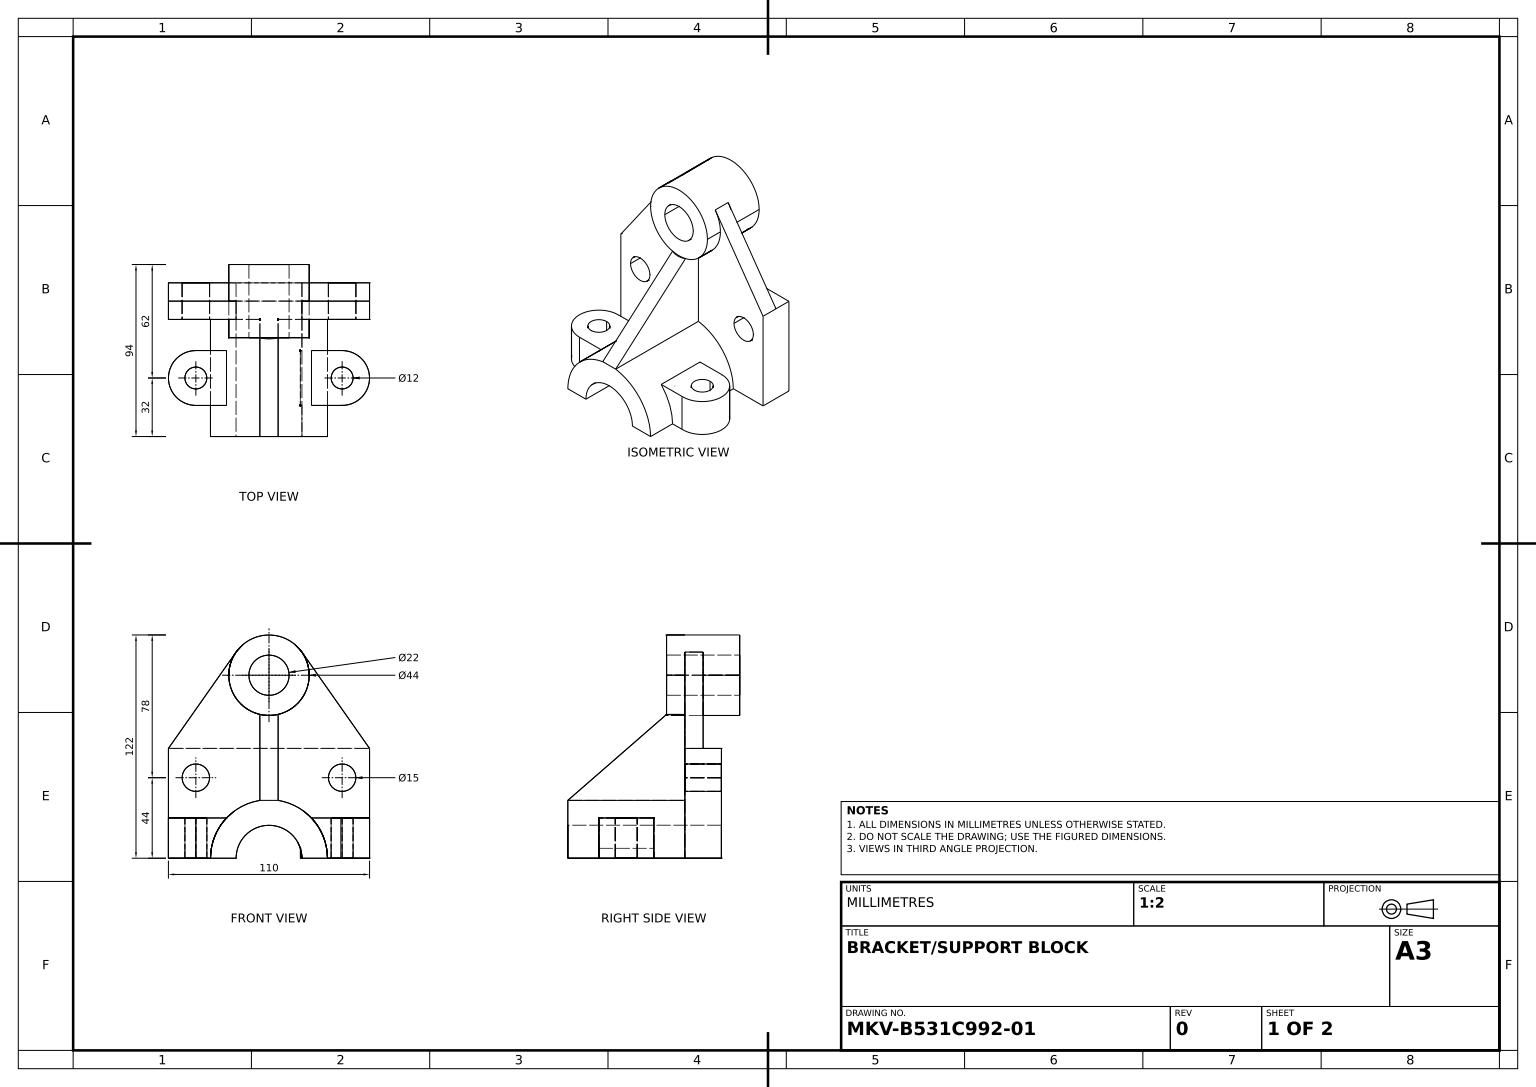
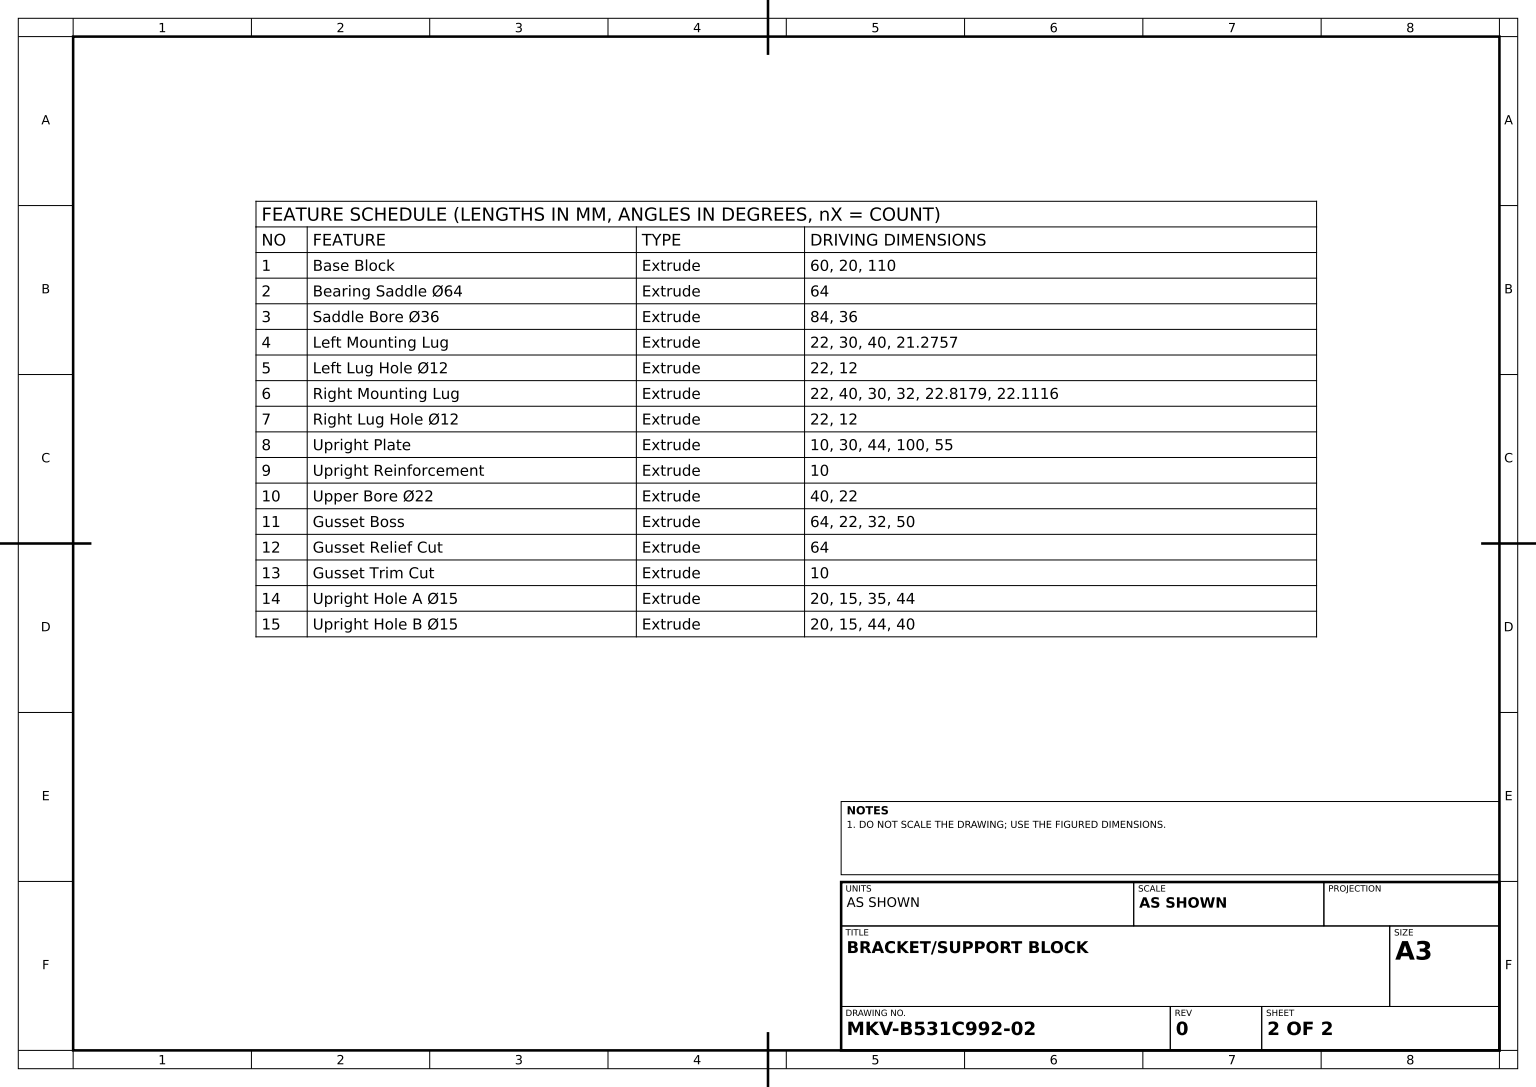
ISO-10303-21;
HEADER;
FILE_DESCRIPTION((''),'2;1');
FILE_NAME('','',(''),(''),'','','');
FILE_SCHEMA(('AUTOMOTIVE_DESIGN'));
ENDSEC;
DATA;
#1=APPLICATION_CONTEXT('');
#2=PRODUCT_CONTEXT('',#1,'mechanical');
#3=PRODUCT('','','',(#2));
#4=PRODUCT_DEFINITION_FORMATION('','',#3);
#5=PRODUCT_DEFINITION_CONTEXT('',#1,'design');
#6=PRODUCT_DEFINITION('','',#4,#5);
#7=PRODUCT_DEFINITION_SHAPE('','',#6);
#8=(LENGTH_UNIT()NAMED_UNIT(*)SI_UNIT(.MILLI.,.METRE.));
#9=(NAMED_UNIT(*)PLANE_ANGLE_UNIT()SI_UNIT($,.RADIAN.));
#10=(NAMED_UNIT(*)SI_UNIT($,.STERADIAN.)SOLID_ANGLE_UNIT());
#11=UNCERTAINTY_MEASURE_WITH_UNIT(LENGTH_MEASURE(1.E-05),#8,'distance_accuracy_value','');
#12=(GEOMETRIC_REPRESENTATION_CONTEXT(3)GLOBAL_UNCERTAINTY_ASSIGNED_CONTEXT((#11))GLOBAL_UNIT_ASSIGNED_CONTEXT((#8,#9,#10))REPRESENTATION_CONTEXT('',''));
#13=CARTESIAN_POINT('',(17.182133,5.364167,17.));
#14=VERTEX_POINT('',#13);
#15=CARTESIAN_POINT('',(17.182133,0.,17.));
#16=VERTEX_POINT('',#15);
#17=CARTESIAN_POINT('',(17.182133,22.,17.));
#18=DIRECTION('',(0.,-1.,0.));
#19=VECTOR('',#18,1000.);
#20=LINE('',#17,#19);
#21=EDGE_CURVE('',#14,#16,#20,.T.);
#22=ORIENTED_EDGE('',*,*,#21,.F.);
#23=CARTESIAN_POINT('',(18.,0.,17.));
#24=VERTEX_POINT('',#23);
#25=CARTESIAN_POINT('',(0.,0.,17.));
#26=DIRECTION('',(0.,0.,-1.));
#27=DIRECTION('',(1.,0.,0.));
#28=AXIS2_PLACEMENT_3D('',#25,#26,#27);
#29=CIRCLE('',#28,18.);
#30=EDGE_CURVE('',#14,#24,#29,.T.);
#31=ORIENTED_EDGE('',*,*,#30,.T.);
#32=CARTESIAN_POINT('',(40.,0.,17.));
#33=DIRECTION('',(-1.,0.,0.));
#34=VECTOR('',#33,1000.);
#35=LINE('',#32,#34);
#36=EDGE_CURVE('',#24,#16,#35,.T.);
#37=ORIENTED_EDGE('',*,*,#36,.T.);
#38=EDGE_LOOP('',(#22,#31,#37));
#39=FACE_OUTER_BOUND('',#38,.T.);
#40=CARTESIAN_POINT('',(40.,22.,17.));
#41=DIRECTION('',(0.,0.,1.));
#42=AXIS2_PLACEMENT_3D('',#40,#41,#27);
#43=PLANE('',#42);
#44=ADVANCED_FACE('',(#39),#43,.F.);
#45=CARTESIAN_POINT('',(-32.,0.,64.));
#46=VERTEX_POINT('',#45);
#47=CARTESIAN_POINT('',(-32.,0.,47.));
#48=VERTEX_POINT('',#47);
#49=VECTOR('',#26,1000.);
#50=LINE('',#45,#49);
#51=EDGE_CURVE('',#46,#48,#50,.T.);
#52=ORIENTED_EDGE('',*,*,#51,.T.);
#53=CARTESIAN_POINT('',(-40.,0.,47.));
#54=VERTEX_POINT('',#53);
#55=CARTESIAN_POINT('',(-18.724275,0.,47.));
#56=VECTOR('',#27,1000.);
#57=LINE('',#55,#56);
#58=EDGE_CURVE('',#54,#48,#57,.T.);
#59=ORIENTED_EDGE('',*,*,#58,.F.);
#60=CARTESIAN_POINT('',(-40.,0.,17.));
#61=VERTEX_POINT('',#60);
#62=CARTESIAN_POINT('',(-40.,0.,32.));
#63=DIRECTION('',(0.,1.,0.));
#64=AXIS2_PLACEMENT_3D('',#62,#63,#41);
#65=CIRCLE('',#64,15.);
#66=EDGE_CURVE('',#61,#54,#65,.T.);
#67=ORIENTED_EDGE('',*,*,#66,.F.);
#68=CARTESIAN_POINT('',(-32.,0.,17.));
#69=VERTEX_POINT('',#68);
#70=LINE('',#60,#34);
#71=EDGE_CURVE('',#69,#61,#70,.T.);
#72=ORIENTED_EDGE('',*,*,#71,.F.);
#73=CARTESIAN_POINT('',(-32.,0.,0.));
#74=VERTEX_POINT('',#73);
#75=EDGE_CURVE('',#69,#74,#50,.T.);
#76=ORIENTED_EDGE('',*,*,#75,.T.);
#77=CARTESIAN_POINT('',(-55.,0.,0.));
#78=VERTEX_POINT('',#77);
#79=CARTESIAN_POINT('',(55.,0.,0.));
#80=LINE('',#79,#56);
#81=EDGE_CURVE('',#78,#74,#80,.T.);
#82=ORIENTED_EDGE('',*,*,#81,.F.);
#83=CARTESIAN_POINT('',(-55.,0.,-20.));
#84=VERTEX_POINT('',#83);
#85=VECTOR('',#41,1000.);
#86=LINE('',#77,#85);
#87=EDGE_CURVE('',#84,#78,#86,.T.);
#88=ORIENTED_EDGE('',*,*,#87,.F.);
#89=CARTESIAN_POINT('',(-18.,0.,-20.));
#90=VERTEX_POINT('',#89);
#91=LINE('',#83,#34);
#92=EDGE_CURVE('',#90,#84,#91,.T.);
#93=ORIENTED_EDGE('',*,*,#92,.F.);
#94=CARTESIAN_POINT('',(-18.,0.,64.));
#95=VERTEX_POINT('',#94);
#96=LINE('',#89,#85);
#97=EDGE_CURVE('',#90,#95,#96,.T.);
#98=ORIENTED_EDGE('',*,*,#97,.T.);
#99=LINE('',#45,#56);
#100=EDGE_CURVE('',#46,#95,#99,.T.);
#101=ORIENTED_EDGE('',*,*,#100,.F.);
#102=EDGE_LOOP('',(#52,#59,#67,#72,#76,#82,#88,#93,#98,#101));
#103=FACE_OUTER_BOUND('',#102,.T.);
#104=CARTESIAN_POINT('',(-40.,0.,26.));
#105=VERTEX_POINT('',#104);
#106=CARTESIAN_POINT('',(-40.,0.,38.));
#107=VERTEX_POINT('',#106);
#108=CIRCLE('',#64,6.);
#109=EDGE_CURVE('',#105,#107,#108,.T.);
#110=ORIENTED_EDGE('',*,*,#109,.T.);
#111=EDGE_CURVE('',#107,#105,#108,.T.);
#112=ORIENTED_EDGE('',*,*,#111,.T.);
#113=EDGE_LOOP('',(#110,#112));
#114=FACE_BOUND('',#113,.T.);
#115=CARTESIAN_POINT('',(0.,0.,0.));
#116=AXIS2_PLACEMENT_3D('',#115,#18,#26);
#117=PLANE('',#116);
#118=ADVANCED_FACE('',(#103,#114),#117,.T.);
#119=CARTESIAN_POINT('',(11.,100.,-30.));
#120=VERTEX_POINT('',#119);
#121=CARTESIAN_POINT('',(-11.,100.,-30.));
#122=VERTEX_POINT('',#121);
#123=CARTESIAN_POINT('',(0.,100.,-30.));
#124=AXIS2_PLACEMENT_3D('',#123,#41,#27);
#125=CIRCLE('',#124,11.);
#126=EDGE_CURVE('',#120,#122,#125,.T.);
#127=ORIENTED_EDGE('',*,*,#126,.F.);
#128=CARTESIAN_POINT('',(11.,100.,10.));
#129=VERTEX_POINT('',#128);
#130=LINE('',#119,#85);
#131=EDGE_CURVE('',#120,#129,#130,.T.);
#132=ORIENTED_EDGE('',*,*,#131,.T.);
#133=CARTESIAN_POINT('',(-11.,100.,10.));
#134=VERTEX_POINT('',#133);
#135=CARTESIAN_POINT('',(0.,100.,10.));
#136=AXIS2_PLACEMENT_3D('',#135,#41,#27);
#137=CIRCLE('',#136,11.);
#138=EDGE_CURVE('',#129,#134,#137,.T.);
#139=ORIENTED_EDGE('',*,*,#138,.T.);
#140=LINE('',#121,#85);
#141=EDGE_CURVE('',#122,#134,#140,.T.);
#142=ORIENTED_EDGE('',*,*,#141,.F.);
#143=EDGE_LOOP('',(#127,#132,#139,#142));
#144=FACE_OUTER_BOUND('',#143,.T.);
#145=CYLINDRICAL_SURFACE('',#124,11.);
#146=ADVANCED_FACE('',(#144),#145,.F.);
#147=CARTESIAN_POINT('',(17.182133,5.364167,47.));
#148=VERTEX_POINT('',#147);
#149=CARTESIAN_POINT('',(17.182133,0.,47.));
#150=VERTEX_POINT('',#149);
#151=CARTESIAN_POINT('',(17.182133,22.,47.));
#152=LINE('',#151,#19);
#153=EDGE_CURVE('',#148,#150,#152,.T.);
#154=ORIENTED_EDGE('',*,*,#153,.T.);
#155=CARTESIAN_POINT('',(18.,0.,46.999385));
#156=VERTEX_POINT('',#155);
#157=DIRECTION('',(0.999999717,0.,-0.000752449));
#158=VECTOR('',#157,1000.);
#159=LINE('',#149,#158);
#160=EDGE_CURVE('',#150,#156,#159,.T.);
#161=ORIENTED_EDGE('',*,*,#160,.T.);
#162=CARTESIAN_POINT('',(18.,1.822601,46.999385));
#163=CARTESIAN_POINT('',(17.725286,3.62438,46.999591));
#164=(BOUNDED_CURVE()B_SPLINE_CURVE(3,(#155,#162,#163,#147),.UNSPECIFIED.,.F.,.T.)B_SPLINE_CURVE_WITH_KNOTS((4,4),(3.141592654,3.444199156),.UNSPECIFIED.)CURVE()GEOMETRIC_REPRESENTATION_ITEM()RATIONAL_B_SPLINE_CURVE((1.,0.992383655,0.992383655,1.))REPRESENTATION_ITEM(''));
#165=EDGE_CURVE('',#156,#148,#164,.T.);
#166=ORIENTED_EDGE('',*,*,#165,.T.);
#167=EDGE_LOOP('',(#154,#161,#166));
#168=FACE_OUTER_BOUND('',#167,.T.);
#169=DIRECTION('',(-0.000752449,0.,-0.999999717));
#170=DIRECTION('',(-0.999999717,0.,0.000752449));
#171=AXIS2_PLACEMENT_3D('',#151,#169,#170);
#172=PLANE('',#171);
#173=ADVANCED_FACE('',(#168),#172,.F.);
#174=CARTESIAN_POINT('',(-40.,22.,47.));
#175=VERTEX_POINT('',#174);
#176=CARTESIAN_POINT('',(-23.2379,22.,47.));
#177=VERTEX_POINT('',#176);
#178=CARTESIAN_POINT('',(-18.724275,22.,47.));
#179=LINE('',#178,#56);
#180=EDGE_CURVE('',#175,#177,#179,.T.);
#181=ORIENTED_EDGE('',*,*,#180,.T.);
#182=CARTESIAN_POINT('',(-23.2379,22.,17.));
#183=VERTEX_POINT('',#182);
#184=CARTESIAN_POINT('',(-23.2379,22.,64.));
#185=LINE('',#184,#85);
#186=EDGE_CURVE('',#183,#177,#185,.T.);
#187=ORIENTED_EDGE('',*,*,#186,.F.);
#188=CARTESIAN_POINT('',(-40.,22.,17.));
#189=VERTEX_POINT('',#188);
#190=LINE('',#188,#34);
#191=EDGE_CURVE('',#183,#189,#190,.T.);
#192=ORIENTED_EDGE('',*,*,#191,.T.);
#193=CARTESIAN_POINT('',(-40.,22.,32.));
#194=AXIS2_PLACEMENT_3D('',#193,#63,#41);
#195=CIRCLE('',#194,15.);
#196=EDGE_CURVE('',#189,#175,#195,.T.);
#197=ORIENTED_EDGE('',*,*,#196,.T.);
#198=EDGE_LOOP('',(#181,#187,#192,#197));
#199=FACE_OUTER_BOUND('',#198,.T.);
#200=CARTESIAN_POINT('',(-40.,22.,26.));
#201=VERTEX_POINT('',#200);
#202=CARTESIAN_POINT('',(-40.,22.,38.));
#203=VERTEX_POINT('',#202);
#204=CIRCLE('',#194,6.);
#205=EDGE_CURVE('',#201,#203,#204,.T.);
#206=ORIENTED_EDGE('',*,*,#205,.F.);
#207=EDGE_CURVE('',#203,#201,#204,.T.);
#208=ORIENTED_EDGE('',*,*,#207,.F.);
#209=EDGE_LOOP('',(#206,#208));
#210=FACE_BOUND('',#209,.T.);
#211=PLANE('',#194);
#212=ADVANCED_FACE('',(#199,#210),#211,.T.);
#213=CARTESIAN_POINT('',(5.,78.575715,10.));
#214=VERTEX_POINT('',#213);
#215=CARTESIAN_POINT('',(22.,100.,10.));
#216=VERTEX_POINT('',#215);
#217=CIRCLE('',#136,22.);
#218=EDGE_CURVE('',#214,#216,#217,.T.);
#219=ORIENTED_EDGE('',*,*,#218,.T.);
#220=CARTESIAN_POINT('',(-22.,100.,10.));
#221=VERTEX_POINT('',#220);
#222=EDGE_CURVE('',#216,#221,#217,.T.);
#223=ORIENTED_EDGE('',*,*,#222,.T.);
#224=CARTESIAN_POINT('',(-5.,78.575715,10.));
#225=VERTEX_POINT('',#224);
#226=EDGE_CURVE('',#221,#225,#217,.T.);
#227=ORIENTED_EDGE('',*,*,#226,.T.);
#228=EDGE_CURVE('',#225,#214,#217,.T.);
#229=ORIENTED_EDGE('',*,*,#228,.T.);
#230=EDGE_LOOP('',(#219,#223,#227,#229));
#231=FACE_OUTER_BOUND('',#230,.T.);
#232=ORIENTED_EDGE('',*,*,#138,.F.);
#233=EDGE_CURVE('',#134,#129,#137,.T.);
#234=ORIENTED_EDGE('',*,*,#233,.F.);
#235=EDGE_LOOP('',(#232,#234));
#236=FACE_BOUND('',#235,.T.);
#237=PLANE('',#136);
#238=ADVANCED_FACE('',(#231,#236),#237,.T.);
#239=CARTESIAN_POINT('',(-55.,60.,-20.));
#240=VERTEX_POINT('',#239);
#241=LINE('',#239,#19);
#242=EDGE_CURVE('',#240,#84,#241,.T.);
#243=ORIENTED_EDGE('',*,*,#242,.F.);
#244=CARTESIAN_POINT('',(55.,60.,-20.));
#245=VERTEX_POINT('',#244);
#246=LINE('',#239,#34);
#247=EDGE_CURVE('',#245,#240,#246,.T.);
#248=ORIENTED_EDGE('',*,*,#247,.F.);
#249=CARTESIAN_POINT('',(55.,0.,-20.));
#250=VERTEX_POINT('',#249);
#251=LINE('',#244,#19);
#252=EDGE_CURVE('',#245,#250,#251,.T.);
#253=ORIENTED_EDGE('',*,*,#252,.T.);
#254=CARTESIAN_POINT('',(18.,0.,-20.));
#255=VERTEX_POINT('',#254);
#256=EDGE_CURVE('',#250,#255,#91,.T.);
#257=ORIENTED_EDGE('',*,*,#256,.T.);
#258=CARTESIAN_POINT('',(0.,0.,-20.));
#259=AXIS2_PLACEMENT_3D('',#258,#41,#27);
#260=CIRCLE('',#259,18.);
#261=EDGE_CURVE('',#255,#90,#260,.T.);
#262=ORIENTED_EDGE('',*,*,#261,.T.);
#263=ORIENTED_EDGE('',*,*,#92,.T.);
#264=EDGE_LOOP('',(#243,#248,#253,#257,#262,#263));
#265=FACE_OUTER_BOUND('',#264,.T.);
#266=CARTESIAN_POINT('',(-47.5,44.,-20.));
#267=VERTEX_POINT('',#266);
#268=CARTESIAN_POINT('',(-32.5,44.,-20.));
#269=VERTEX_POINT('',#268);
#270=CARTESIAN_POINT('',(-40.,44.,-20.));
#271=AXIS2_PLACEMENT_3D('',#270,#41,#27);
#272=CIRCLE('',#271,7.5);
#273=EDGE_CURVE('',#267,#269,#272,.T.);
#274=ORIENTED_EDGE('',*,*,#273,.T.);
#275=EDGE_CURVE('',#269,#267,#272,.T.);
#276=ORIENTED_EDGE('',*,*,#275,.T.);
#277=EDGE_LOOP('',(#274,#276));
#278=FACE_BOUND('',#277,.T.);
#279=CARTESIAN_POINT('',(47.5,44.,-20.));
#280=VERTEX_POINT('',#279);
#281=CARTESIAN_POINT('',(32.5,44.,-20.));
#282=VERTEX_POINT('',#281);
#283=CARTESIAN_POINT('',(40.,44.,-20.));
#284=AXIS2_PLACEMENT_3D('',#283,#41,#27);
#285=CIRCLE('',#284,7.5);
#286=EDGE_CURVE('',#280,#282,#285,.T.);
#287=ORIENTED_EDGE('',*,*,#286,.T.);
#288=EDGE_CURVE('',#282,#280,#285,.T.);
#289=ORIENTED_EDGE('',*,*,#288,.T.);
#290=EDGE_LOOP('',(#287,#289));
#291=FACE_BOUND('',#290,.T.);
#292=AXIS2_PLACEMENT_3D('',#239,#41,#27);
#293=PLANE('',#292);
#294=ADVANCED_FACE('',(#265,#278,#291),#293,.F.);
#295=ORIENTED_EDGE('',*,*,#131,.F.);
#296=EDGE_CURVE('',#122,#120,#125,.T.);
#297=ORIENTED_EDGE('',*,*,#296,.F.);
#298=ORIENTED_EDGE('',*,*,#141,.T.);
#299=ORIENTED_EDGE('',*,*,#233,.T.);
#300=EDGE_LOOP('',(#295,#297,#298,#299));
#301=FACE_OUTER_BOUND('',#300,.T.);
#302=ADVANCED_FACE('',(#301),#145,.F.);
#303=CARTESIAN_POINT('',(-5.,31.606961,64.));
#304=VERTEX_POINT('',#303);
#305=CARTESIAN_POINT('',(-5.,51.83632,40.742296));
#306=DIRECTION('',(0.,0.65627603,-0.754520889));
#307=VECTOR('',#306,1000.);
#308=LINE('',#305,#307);
#309=EDGE_CURVE('',#304,#225,#308,.T.);
#310=ORIENTED_EDGE('',*,*,#309,.F.);
#311=CARTESIAN_POINT('',(5.,31.606961,64.));
#312=VERTEX_POINT('',#311);
#313=CARTESIAN_POINT('',(-64.,31.606961,64.));
#314=LINE('',#313,#56);
#315=EDGE_CURVE('',#304,#312,#314,.T.);
#316=ORIENTED_EDGE('',*,*,#315,.T.);
#317=CARTESIAN_POINT('',(5.,51.83632,40.742296));
#318=DIRECTION('',(0.,-0.65627603,0.754520889));
#319=VECTOR('',#318,1000.);
#320=LINE('',#317,#319);
#321=EDGE_CURVE('',#214,#312,#320,.T.);
#322=ORIENTED_EDGE('',*,*,#321,.F.);
#323=CARTESIAN_POINT('',(-1.696259,77.804688,10.88645));
#324=CARTESIAN_POINT('',(1.696259,77.804688,10.88645));
#325=(BOUNDED_CURVE()B_SPLINE_CURVE(3,(#224,#323,#324,#213),.UNSPECIFIED.,.F.,.T.)B_SPLINE_CURVE_WITH_KNOTS((4,4),(2.91231645,3.370868857),.UNSPECIFIED.)CURVE()GEOMETRIC_REPRESENTATION_ITEM()RATIONAL_B_SPLINE_CURVE((1.,0.9825541,0.9825541,1.))REPRESENTATION_ITEM(''));
#326=EDGE_CURVE('',#225,#214,#325,.T.);
#327=ORIENTED_EDGE('',*,*,#326,.F.);
#328=EDGE_LOOP('',(#310,#316,#322,#327));
#329=FACE_OUTER_BOUND('',#328,.T.);
#330=CARTESIAN_POINT('',(-64.,78.575715,10.));
#331=DIRECTION('',(0.,-0.754520889,-0.65627603));
#332=AXIS2_PLACEMENT_3D('',#330,#331,#306);
#333=PLANE('',#332);
#334=ADVANCED_FACE('',(#329),#333,.F.);
#335=CARTESIAN_POINT('',(40.,22.,26.));
#336=VERTEX_POINT('',#335);
#337=CARTESIAN_POINT('',(40.,22.,38.));
#338=VERTEX_POINT('',#337);
#339=CARTESIAN_POINT('',(40.,22.,32.));
#340=AXIS2_PLACEMENT_3D('',#339,#63,#41);
#341=CIRCLE('',#340,6.);
#342=EDGE_CURVE('',#336,#338,#341,.T.);
#343=ORIENTED_EDGE('',*,*,#342,.T.);
#344=CARTESIAN_POINT('',(40.,0.,38.));
#345=VERTEX_POINT('',#344);
#346=VECTOR('',#63,1000.);
#347=LINE('',#344,#346);
#348=EDGE_CURVE('',#345,#338,#347,.T.);
#349=ORIENTED_EDGE('',*,*,#348,.F.);
#350=CARTESIAN_POINT('',(40.,0.,26.));
#351=VERTEX_POINT('',#350);
#352=CARTESIAN_POINT('',(40.,0.,32.));
#353=AXIS2_PLACEMENT_3D('',#352,#63,#41);
#354=CIRCLE('',#353,6.);
#355=EDGE_CURVE('',#351,#345,#354,.T.);
#356=ORIENTED_EDGE('',*,*,#355,.F.);
#357=LINE('',#350,#346);
#358=EDGE_CURVE('',#351,#336,#357,.T.);
#359=ORIENTED_EDGE('',*,*,#358,.T.);
#360=EDGE_LOOP('',(#343,#349,#356,#359));
#361=FACE_OUTER_BOUND('',#360,.T.);
#362=CYLINDRICAL_SURFACE('',#353,6.);
#363=ADVANCED_FACE('',(#361),#362,.F.);
#364=AXIS2_PLACEMENT_3D('',#25,#41,#27);
#365=CIRCLE('',#364,32.);
#366=EDGE_CURVE('',#183,#69,#365,.T.);
#367=ORIENTED_EDGE('',*,*,#366,.T.);
#368=ORIENTED_EDGE('',*,*,#71,.T.);
#369=LINE('',#188,#19);
#370=EDGE_CURVE('',#189,#61,#369,.T.);
#371=ORIENTED_EDGE('',*,*,#370,.F.);
#372=ORIENTED_EDGE('',*,*,#191,.F.);
#373=EDGE_LOOP('',(#367,#368,#371,#372));
#374=FACE_OUTER_BOUND('',#373,.T.);
#375=AXIS2_PLACEMENT_3D('',#188,#41,#27);
#376=PLANE('',#375);
#377=ADVANCED_FACE('',(#374),#376,.F.);
#378=VERTEX_POINT('',#32);
#379=CARTESIAN_POINT('',(32.,0.,17.));
#380=VERTEX_POINT('',#379);
#381=EDGE_CURVE('',#378,#380,#35,.T.);
#382=ORIENTED_EDGE('',*,*,#381,.T.);
#383=CARTESIAN_POINT('',(23.2379,22.,17.));
#384=VERTEX_POINT('',#383);
#385=EDGE_CURVE('',#380,#384,#365,.T.);
#386=ORIENTED_EDGE('',*,*,#385,.T.);
#387=VERTEX_POINT('',#40);
#388=LINE('',#40,#34);
#389=EDGE_CURVE('',#387,#384,#388,.T.);
#390=ORIENTED_EDGE('',*,*,#389,.F.);
#391=LINE('',#40,#19);
#392=EDGE_CURVE('',#387,#378,#391,.T.);
#393=ORIENTED_EDGE('',*,*,#392,.T.);
#394=EDGE_LOOP('',(#382,#386,#390,#393));
#395=FACE_OUTER_BOUND('',#394,.T.);
#396=ADVANCED_FACE('',(#395),#43,.F.);
#397=ORIENTED_EDGE('',*,*,#273,.F.);
#398=CARTESIAN_POINT('',(-47.5,44.,0.));
#399=VERTEX_POINT('',#398);
#400=LINE('',#266,#85);
#401=EDGE_CURVE('',#267,#399,#400,.T.);
#402=ORIENTED_EDGE('',*,*,#401,.T.);
#403=CARTESIAN_POINT('',(-32.5,44.,0.));
#404=VERTEX_POINT('',#403);
#405=CARTESIAN_POINT('',(-40.,44.,0.));
#406=AXIS2_PLACEMENT_3D('',#405,#41,#27);
#407=CIRCLE('',#406,7.5);
#408=EDGE_CURVE('',#399,#404,#407,.T.);
#409=ORIENTED_EDGE('',*,*,#408,.T.);
#410=LINE('',#268,#85);
#411=EDGE_CURVE('',#269,#404,#410,.T.);
#412=ORIENTED_EDGE('',*,*,#411,.F.);
#413=EDGE_LOOP('',(#397,#402,#409,#412));
#414=FACE_OUTER_BOUND('',#413,.T.);
#415=CYLINDRICAL_SURFACE('',#271,7.5);
#416=ADVANCED_FACE('',(#414),#415,.F.);
#417=CARTESIAN_POINT('',(22.,100.,-30.));
#418=VERTEX_POINT('',#417);
#419=CARTESIAN_POINT('',(22.,100.,-10.));
#420=VERTEX_POINT('',#419);
#421=LINE('',#417,#85);
#422=EDGE_CURVE('',#418,#420,#421,.T.);
#423=ORIENTED_EDGE('',*,*,#422,.F.);
#424=CARTESIAN_POINT('',(-22.,100.,-30.));
#425=VERTEX_POINT('',#424);
#426=CIRCLE('',#124,22.);
#427=EDGE_CURVE('',#418,#425,#426,.T.);
#428=ORIENTED_EDGE('',*,*,#427,.T.);
#429=CARTESIAN_POINT('',(-22.,100.,-10.));
#430=VERTEX_POINT('',#429);
#431=LINE('',#424,#85);
#432=EDGE_CURVE('',#425,#430,#431,.T.);
#433=ORIENTED_EDGE('',*,*,#432,.T.);
#434=CARTESIAN_POINT('',(-17.999682,112.649563,-10.));
#435=VERTEX_POINT('',#434);
#436=CARTESIAN_POINT('',(0.,100.,-10.));
#437=AXIS2_PLACEMENT_3D('',#436,#26,#27);
#438=CIRCLE('',#437,22.);
#439=EDGE_CURVE('',#430,#435,#438,.T.);
#440=ORIENTED_EDGE('',*,*,#439,.T.);
#441=CARTESIAN_POINT('',(-17.999682,112.649563,0.));
#442=VERTEX_POINT('',#441);
#443=LINE('',#434,#85);
#444=EDGE_CURVE('',#435,#442,#443,.T.);
#445=ORIENTED_EDGE('',*,*,#444,.T.);
#446=CARTESIAN_POINT('',(-22.,100.,0.));
#447=VERTEX_POINT('',#446);
#448=CARTESIAN_POINT('',(0.,100.,0.));
#449=AXIS2_PLACEMENT_3D('',#448,#26,#27);
#450=CIRCLE('',#449,22.);
#451=EDGE_CURVE('',#447,#442,#450,.T.);
#452=ORIENTED_EDGE('',*,*,#451,.F.);
#453=EDGE_CURVE('',#447,#221,#431,.T.);
#454=ORIENTED_EDGE('',*,*,#453,.T.);
#455=ORIENTED_EDGE('',*,*,#222,.F.);
#456=CARTESIAN_POINT('',(22.,100.,0.));
#457=VERTEX_POINT('',#456);
#458=EDGE_CURVE('',#457,#216,#421,.T.);
#459=ORIENTED_EDGE('',*,*,#458,.F.);
#460=CARTESIAN_POINT('',(17.999682,112.649563,0.));
#461=VERTEX_POINT('',#460);
#462=EDGE_CURVE('',#461,#457,#450,.T.);
#463=ORIENTED_EDGE('',*,*,#462,.F.);
#464=CARTESIAN_POINT('',(17.999682,112.649563,-10.));
#465=VERTEX_POINT('',#464);
#466=LINE('',#464,#85);
#467=EDGE_CURVE('',#465,#461,#466,.T.);
#468=ORIENTED_EDGE('',*,*,#467,.F.);
#469=EDGE_CURVE('',#465,#420,#438,.T.);
#470=ORIENTED_EDGE('',*,*,#469,.T.);
#471=EDGE_LOOP('',(#423,#428,#433,#440,#445,#452,#454,#455,#459,#463,#468,#470));
#472=FACE_OUTER_BOUND('',#471,.T.);
#473=CYLINDRICAL_SURFACE('',#124,22.);
#474=ADVANCED_FACE('',(#472),#473,.T.);
#475=ORIENTED_EDGE('',*,*,#207,.T.);
#476=LINE('',#104,#346);
#477=EDGE_CURVE('',#105,#201,#476,.T.);
#478=ORIENTED_EDGE('',*,*,#477,.F.);
#479=ORIENTED_EDGE('',*,*,#111,.F.);
#480=LINE('',#106,#346);
#481=EDGE_CURVE('',#107,#203,#480,.T.);
#482=ORIENTED_EDGE('',*,*,#481,.T.);
#483=EDGE_LOOP('',(#475,#478,#479,#482));
#484=FACE_OUTER_BOUND('',#483,.T.);
#485=CYLINDRICAL_SURFACE('',#64,6.);
#486=ADVANCED_FACE('',(#484),#485,.F.);
#487=ORIENTED_EDGE('',*,*,#218,.F.);
#488=CARTESIAN_POINT('',(5.,78.575715,0.));
#489=VERTEX_POINT('',#488);
#490=CARTESIAN_POINT('',(5.,78.575715,64.));
#491=LINE('',#490,#49);
#492=EDGE_CURVE('',#214,#489,#491,.T.);
#493=ORIENTED_EDGE('',*,*,#492,.T.);
#494=EDGE_CURVE('',#457,#489,#450,.T.);
#495=ORIENTED_EDGE('',*,*,#494,.F.);
#496=ORIENTED_EDGE('',*,*,#458,.T.);
#497=EDGE_LOOP('',(#487,#493,#495,#496));
#498=FACE_OUTER_BOUND('',#497,.T.);
#499=ADVANCED_FACE('',(#498),#473,.T.);
#500=CARTESIAN_POINT('',(-5.,78.575715,0.));
#501=VERTEX_POINT('',#500);
#502=CARTESIAN_POINT('',(-5.,78.575715,64.));
#503=LINE('',#502,#49);
#504=EDGE_CURVE('',#225,#501,#503,.T.);
#505=ORIENTED_EDGE('',*,*,#504,.T.);
#506=CARTESIAN_POINT('',(-5.,31.606961,0.));
#507=VERTEX_POINT('',#506);
#508=LINE('',#500,#19);
#509=EDGE_CURVE('',#501,#507,#508,.T.);
#510=ORIENTED_EDGE('',*,*,#509,.T.);
#511=LINE('',#303,#49);
#512=EDGE_CURVE('',#304,#507,#511,.T.);
#513=ORIENTED_EDGE('',*,*,#512,.F.);
#514=ORIENTED_EDGE('',*,*,#309,.T.);
#515=EDGE_LOOP('',(#505,#510,#513,#514));
#516=FACE_OUTER_BOUND('',#515,.T.);
#517=AXIS2_PLACEMENT_3D('',#502,#27,#26);
#518=PLANE('',#517);
#519=ADVANCED_FACE('',(#516),#518,.F.);
#520=ORIENTED_EDGE('',*,*,#392,.F.);
#521=CARTESIAN_POINT('',(39.293701,22.,46.983362));
#522=VERTEX_POINT('',#521);
#523=CIRCLE('',#340,15.);
#524=EDGE_CURVE('',#522,#387,#523,.T.);
#525=ORIENTED_EDGE('',*,*,#524,.F.);
#526=CARTESIAN_POINT('',(39.293701,0.,46.983362));
#527=VERTEX_POINT('',#526);
#528=LINE('',#521,#19);
#529=EDGE_CURVE('',#522,#527,#528,.T.);
#530=ORIENTED_EDGE('',*,*,#529,.T.);
#531=CIRCLE('',#353,15.);
#532=EDGE_CURVE('',#527,#378,#531,.T.);
#533=ORIENTED_EDGE('',*,*,#532,.T.);
#534=EDGE_LOOP('',(#520,#525,#530,#533));
#535=FACE_OUTER_BOUND('',#534,.T.);
#536=AXIS2_PLACEMENT_3D('',#339,#18,#26);
#537=CYLINDRICAL_SURFACE('',#536,15.);
#538=ADVANCED_FACE('',(#535),#537,.T.);
#539=ORIENTED_EDGE('',*,*,#477,.T.);
#540=ORIENTED_EDGE('',*,*,#205,.T.);
#541=ORIENTED_EDGE('',*,*,#481,.F.);
#542=ORIENTED_EDGE('',*,*,#109,.F.);
#543=EDGE_LOOP('',(#539,#540,#541,#542));
#544=FACE_OUTER_BOUND('',#543,.T.);
#545=ADVANCED_FACE('',(#544),#485,.F.);
#546=ORIENTED_EDGE('',*,*,#467,.T.);
#547=CARTESIAN_POINT('',(55.,60.,0.));
#548=VERTEX_POINT('',#547);
#549=DIRECTION('',(-0.574980134,0.81816737,0.));
#550=VECTOR('',#549,1000.);
#551=LINE('',#547,#550);
#552=EDGE_CURVE('',#548,#461,#551,.T.);
#553=ORIENTED_EDGE('',*,*,#552,.F.);
#554=CARTESIAN_POINT('',(55.,60.,-10.));
#555=VERTEX_POINT('',#554);
#556=LINE('',#244,#49);
#557=EDGE_CURVE('',#548,#555,#556,.T.);
#558=ORIENTED_EDGE('',*,*,#557,.T.);
#559=LINE('',#554,#550);
#560=EDGE_CURVE('',#555,#465,#559,.T.);
#561=ORIENTED_EDGE('',*,*,#560,.T.);
#562=EDGE_LOOP('',(#546,#553,#558,#561));
#563=FACE_OUTER_BOUND('',#562,.T.);
#564=DIRECTION('',(0.81816737,0.574980134,0.));
#565=AXIS2_PLACEMENT_3D('',#554,#564,#549);
#566=PLANE('',#565);
#567=ADVANCED_FACE('',(#563),#566,.T.);
#568=ORIENTED_EDGE('',*,*,#444,.F.);
#569=CARTESIAN_POINT('',(-55.,60.,-10.));
#570=VERTEX_POINT('',#569);
#571=DIRECTION('',(-0.574980134,-0.81816737,0.));
#572=VECTOR('',#571,1000.);
#573=LINE('',#569,#572);
#574=EDGE_CURVE('',#435,#570,#573,.T.);
#575=ORIENTED_EDGE('',*,*,#574,.T.);
#576=CARTESIAN_POINT('',(-55.,60.,0.));
#577=VERTEX_POINT('',#576);
#578=LINE('',#569,#85);
#579=EDGE_CURVE('',#570,#577,#578,.T.);
#580=ORIENTED_EDGE('',*,*,#579,.T.);
#581=LINE('',#576,#572);
#582=EDGE_CURVE('',#442,#577,#581,.T.);
#583=ORIENTED_EDGE('',*,*,#582,.F.);
#584=EDGE_LOOP('',(#568,#575,#580,#583));
#585=FACE_OUTER_BOUND('',#584,.T.);
#586=DIRECTION('',(-0.81816737,0.574980134,0.));
#587=AXIS2_PLACEMENT_3D('',#569,#586,#571);
#588=PLANE('',#587);
#589=ADVANCED_FACE('',(#585),#588,.T.);
#590=ORIENTED_EDGE('',*,*,#366,.F.);
#591=ORIENTED_EDGE('',*,*,#186,.T.);
#592=CARTESIAN_POINT('',(0.,0.,47.));
#593=AXIS2_PLACEMENT_3D('',#592,#26,#33);
#594=CIRCLE('',#593,32.);
#595=EDGE_CURVE('',#48,#177,#594,.T.);
#596=ORIENTED_EDGE('',*,*,#595,.F.);
#597=ORIENTED_EDGE('',*,*,#51,.F.);
#598=CARTESIAN_POINT('',(0.,0.,64.));
#599=AXIS2_PLACEMENT_3D('',#598,#41,#27);
#600=CIRCLE('',#599,32.);
#601=EDGE_CURVE('',#304,#46,#600,.T.);
#602=ORIENTED_EDGE('',*,*,#601,.F.);
#603=ORIENTED_EDGE('',*,*,#512,.T.);
#604=AXIS2_PLACEMENT_3D('',#115,#41,#27);
#605=CIRCLE('',#604,32.);
#606=EDGE_CURVE('',#507,#74,#605,.T.);
#607=ORIENTED_EDGE('',*,*,#606,.T.);
#608=ORIENTED_EDGE('',*,*,#75,.F.);
#609=EDGE_LOOP('',(#590,#591,#596,#597,#602,#603,#607,#608));
#610=FACE_OUTER_BOUND('',#609,.T.);
#611=AXIS2_PLACEMENT_3D('',#598,#26,#33);
#612=CYLINDRICAL_SURFACE('',#611,32.);
#613=ADVANCED_FACE('',(#610),#612,.T.);
#614=LINE('',#569,#56);
#615=EDGE_CURVE('',#570,#555,#614,.T.);
#616=ORIENTED_EDGE('',*,*,#615,.F.);
#617=ORIENTED_EDGE('',*,*,#574,.F.);
#618=ORIENTED_EDGE('',*,*,#439,.F.);
#619=EDGE_CURVE('',#420,#430,#438,.T.);
#620=ORIENTED_EDGE('',*,*,#619,.F.);
#621=ORIENTED_EDGE('',*,*,#469,.F.);
#622=ORIENTED_EDGE('',*,*,#560,.F.);
#623=EDGE_LOOP('',(#616,#617,#618,#620,#621,#622));
#624=FACE_OUTER_BOUND('',#623,.T.);
#625=AXIS2_PLACEMENT_3D('',#436,#41,#27);
#626=PLANE('',#625);
#627=ADVANCED_FACE('',(#624),#626,.F.);
#628=ORIENTED_EDGE('',*,*,#288,.F.);
#629=CARTESIAN_POINT('',(32.5,44.,0.));
#630=VERTEX_POINT('',#629);
#631=LINE('',#281,#85);
#632=EDGE_CURVE('',#282,#630,#631,.T.);
#633=ORIENTED_EDGE('',*,*,#632,.T.);
#634=CARTESIAN_POINT('',(47.5,44.,0.));
#635=VERTEX_POINT('',#634);
#636=CARTESIAN_POINT('',(40.,44.,0.));
#637=AXIS2_PLACEMENT_3D('',#636,#41,#27);
#638=CIRCLE('',#637,7.5);
#639=EDGE_CURVE('',#630,#635,#638,.T.);
#640=ORIENTED_EDGE('',*,*,#639,.T.);
#641=LINE('',#279,#85);
#642=EDGE_CURVE('',#280,#635,#641,.T.);
#643=ORIENTED_EDGE('',*,*,#642,.F.);
#644=EDGE_LOOP('',(#628,#633,#640,#643));
#645=FACE_OUTER_BOUND('',#644,.T.);
#646=CYLINDRICAL_SURFACE('',#284,7.5);
#647=ADVANCED_FACE('',(#645),#646,.F.);
#648=ORIENTED_EDGE('',*,*,#422,.T.);
#649=ORIENTED_EDGE('',*,*,#619,.T.);
#650=ORIENTED_EDGE('',*,*,#432,.F.);
#651=EDGE_CURVE('',#425,#418,#426,.T.);
#652=ORIENTED_EDGE('',*,*,#651,.T.);
#653=EDGE_LOOP('',(#648,#649,#650,#652));
#654=FACE_OUTER_BOUND('',#653,.T.);
#655=ADVANCED_FACE('',(#654),#473,.T.);
#656=EDGE_CURVE('',#345,#351,#354,.T.);
#657=ORIENTED_EDGE('',*,*,#656,.T.);
#658=ORIENTED_EDGE('',*,*,#355,.T.);
#659=EDGE_LOOP('',(#657,#658));
#660=FACE_BOUND('',#659,.T.);
#661=CARTESIAN_POINT('',(32.,0.,0.));
#662=VERTEX_POINT('',#661);
#663=CARTESIAN_POINT('',(32.,0.,64.));
#664=LINE('',#663,#49);
#665=EDGE_CURVE('',#380,#662,#664,.T.);
#666=ORIENTED_EDGE('',*,*,#665,.F.);
#667=ORIENTED_EDGE('',*,*,#381,.F.);
#668=ORIENTED_EDGE('',*,*,#532,.F.);
#669=CARTESIAN_POINT('',(32.,0.,46.98885));
#670=VERTEX_POINT('',#669);
#671=EDGE_CURVE('',#670,#527,#159,.T.);
#672=ORIENTED_EDGE('',*,*,#671,.F.);
#673=VERTEX_POINT('',#663);
#674=EDGE_CURVE('',#673,#670,#664,.T.);
#675=ORIENTED_EDGE('',*,*,#674,.F.);
#676=CARTESIAN_POINT('',(18.,0.,64.));
#677=VERTEX_POINT('',#676);
#678=EDGE_CURVE('',#677,#673,#99,.T.);
#679=ORIENTED_EDGE('',*,*,#678,.F.);
#680=LINE('',#254,#85);
#681=EDGE_CURVE('',#156,#677,#680,.T.);
#682=ORIENTED_EDGE('',*,*,#681,.F.);
#683=ORIENTED_EDGE('',*,*,#160,.F.);
#684=LINE('',#15,#85);
#685=EDGE_CURVE('',#16,#150,#684,.T.);
#686=ORIENTED_EDGE('',*,*,#685,.F.);
#687=ORIENTED_EDGE('',*,*,#36,.F.);
#688=EDGE_CURVE('',#255,#24,#680,.T.);
#689=ORIENTED_EDGE('',*,*,#688,.F.);
#690=ORIENTED_EDGE('',*,*,#256,.F.);
#691=VERTEX_POINT('',#79);
#692=LINE('',#249,#49);
#693=EDGE_CURVE('',#691,#250,#692,.T.);
#694=ORIENTED_EDGE('',*,*,#693,.F.);
#695=EDGE_CURVE('',#662,#691,#80,.T.);
#696=ORIENTED_EDGE('',*,*,#695,.F.);
#697=EDGE_LOOP('',(#666,#667,#668,#672,#675,#679,#682,#683,#686,#687,#689,#690,#694,#696));
#698=FACE_OUTER_BOUND('',#697,.T.);
#699=ADVANCED_FACE('',(#660,#698),#117,.T.);
#700=ORIENTED_EDGE('',*,*,#87,.T.);
#701=LINE('',#576,#19);
#702=EDGE_CURVE('',#577,#78,#701,.T.);
#703=ORIENTED_EDGE('',*,*,#702,.F.);
#704=ORIENTED_EDGE('',*,*,#579,.F.);
#705=LINE('',#576,#85);
#706=EDGE_CURVE('',#240,#570,#705,.T.);
#707=ORIENTED_EDGE('',*,*,#706,.F.);
#708=ORIENTED_EDGE('',*,*,#242,.T.);
#709=EDGE_LOOP('',(#700,#703,#704,#707,#708));
#710=FACE_OUTER_BOUND('',#709,.T.);
#711=AXIS2_PLACEMENT_3D('',#576,#27,#26);
#712=PLANE('',#711);
#713=ADVANCED_FACE('',(#710),#712,.F.);
#714=ORIENTED_EDGE('',*,*,#632,.F.);
#715=ORIENTED_EDGE('',*,*,#286,.F.);
#716=ORIENTED_EDGE('',*,*,#642,.T.);
#717=EDGE_CURVE('',#635,#630,#638,.T.);
#718=ORIENTED_EDGE('',*,*,#717,.T.);
#719=EDGE_LOOP('',(#714,#715,#716,#718));
#720=FACE_OUTER_BOUND('',#719,.T.);
#721=ADVANCED_FACE('',(#720),#646,.F.);
#722=ORIENTED_EDGE('',*,*,#504,.F.);
#723=ORIENTED_EDGE('',*,*,#226,.F.);
#724=ORIENTED_EDGE('',*,*,#453,.F.);
#725=EDGE_CURVE('',#501,#447,#450,.T.);
#726=ORIENTED_EDGE('',*,*,#725,.F.);
#727=EDGE_LOOP('',(#722,#723,#724,#726));
#728=FACE_OUTER_BOUND('',#727,.T.);
#729=ADVANCED_FACE('',(#728),#473,.T.);
#730=ORIENTED_EDGE('',*,*,#408,.F.);
#731=EDGE_CURVE('',#404,#399,#407,.T.);
#732=ORIENTED_EDGE('',*,*,#731,.F.);
#733=EDGE_LOOP('',(#730,#732));
#734=FACE_BOUND('',#733,.T.);
#735=ORIENTED_EDGE('',*,*,#606,.F.);
#736=ORIENTED_EDGE('',*,*,#509,.F.);
#737=ORIENTED_EDGE('',*,*,#725,.T.);
#738=ORIENTED_EDGE('',*,*,#451,.T.);
#739=ORIENTED_EDGE('',*,*,#582,.T.);
#740=ORIENTED_EDGE('',*,*,#702,.T.);
#741=ORIENTED_EDGE('',*,*,#81,.T.);
#742=EDGE_LOOP('',(#735,#736,#737,#738,#739,#740,#741));
#743=FACE_OUTER_BOUND('',#742,.T.);
#744=AXIS2_PLACEMENT_3D('',#547,#26,#33);
#745=PLANE('',#744);
#746=ADVANCED_FACE('',(#734,#743),#745,.F.);
#747=ORIENTED_EDGE('',*,*,#557,.F.);
#748=LINE('',#547,#19);
#749=EDGE_CURVE('',#548,#691,#748,.T.);
#750=ORIENTED_EDGE('',*,*,#749,.T.);
#751=ORIENTED_EDGE('',*,*,#693,.T.);
#752=ORIENTED_EDGE('',*,*,#252,.F.);
#753=EDGE_CURVE('',#555,#245,#556,.T.);
#754=ORIENTED_EDGE('',*,*,#753,.F.);
#755=EDGE_LOOP('',(#747,#750,#751,#752,#754));
#756=FACE_OUTER_BOUND('',#755,.T.);
#757=AXIS2_PLACEMENT_3D('',#244,#33,#41);
#758=PLANE('',#757);
#759=ADVANCED_FACE('',(#756),#758,.F.);
#760=ORIENTED_EDGE('',*,*,#385,.F.);
#761=ORIENTED_EDGE('',*,*,#665,.T.);
#762=CARTESIAN_POINT('',(5.,31.606961,0.));
#763=VERTEX_POINT('',#762);
#764=EDGE_CURVE('',#662,#763,#605,.T.);
#765=ORIENTED_EDGE('',*,*,#764,.T.);
#766=LINE('',#311,#49);
#767=EDGE_CURVE('',#312,#763,#766,.T.);
#768=ORIENTED_EDGE('',*,*,#767,.F.);
#769=EDGE_CURVE('',#673,#312,#600,.T.);
#770=ORIENTED_EDGE('',*,*,#769,.F.);
#771=ORIENTED_EDGE('',*,*,#674,.T.);
#772=CARTESIAN_POINT('',(23.2379,22.,46.995443));
#773=VERTEX_POINT('',#772);
#774=CARTESIAN_POINT('',(28.934244,15.983133,46.991157));
#775=CARTESIAN_POINT('',(32.,8.285591,46.98885));
#776=(BOUNDED_CURVE()B_SPLINE_CURVE(3,(#772,#774,#775,#669),.UNSPECIFIED.,.F.,.T.)B_SPLINE_CURVE_WITH_KNOTS((4,4),(5.525144542,6.283185307),.UNSPECIFIED.)CURVE()GEOMETRIC_REPRESENTATION_ITEM()RATIONAL_B_SPLINE_CURVE((1.,0.952685033,0.952685033,1.))REPRESENTATION_ITEM(''));
#777=EDGE_CURVE('',#773,#670,#776,.T.);
#778=ORIENTED_EDGE('',*,*,#777,.F.);
#779=CARTESIAN_POINT('',(23.2379,22.,64.));
#780=LINE('',#779,#49);
#781=EDGE_CURVE('',#773,#384,#780,.T.);
#782=ORIENTED_EDGE('',*,*,#781,.T.);
#783=EDGE_LOOP('',(#760,#761,#765,#768,#770,#771,#778,#782));
#784=FACE_OUTER_BOUND('',#783,.T.);
#785=ADVANCED_FACE('',(#784),#612,.T.);
#786=ORIENTED_EDGE('',*,*,#681,.T.);
#787=CIRCLE('',#599,18.);
#788=EDGE_CURVE('',#677,#95,#787,.T.);
#789=ORIENTED_EDGE('',*,*,#788,.T.);
#790=ORIENTED_EDGE('',*,*,#97,.F.);
#791=ORIENTED_EDGE('',*,*,#261,.F.);
#792=ORIENTED_EDGE('',*,*,#688,.T.);
#793=ORIENTED_EDGE('',*,*,#30,.F.);
#794=CARTESIAN_POINT('',(17.182133,5.364167,-20.));
#795=LINE('',#794,#49);
#796=EDGE_CURVE('',#148,#14,#795,.T.);
#797=ORIENTED_EDGE('',*,*,#796,.F.);
#798=ORIENTED_EDGE('',*,*,#165,.F.);
#799=EDGE_LOOP('',(#786,#789,#790,#791,#792,#793,#797,#798));
#800=FACE_OUTER_BOUND('',#799,.T.);
#801=CYLINDRICAL_SURFACE('',#259,18.);
#802=ADVANCED_FACE('',(#800),#801,.F.);
#803=ORIENTED_EDGE('',*,*,#764,.F.);
#804=ORIENTED_EDGE('',*,*,#695,.T.);
#805=ORIENTED_EDGE('',*,*,#749,.F.);
#806=ORIENTED_EDGE('',*,*,#552,.T.);
#807=ORIENTED_EDGE('',*,*,#462,.T.);
#808=ORIENTED_EDGE('',*,*,#494,.T.);
#809=LINE('',#488,#346);
#810=EDGE_CURVE('',#763,#489,#809,.T.);
#811=ORIENTED_EDGE('',*,*,#810,.F.);
#812=EDGE_LOOP('',(#803,#804,#805,#806,#807,#808,#811));
#813=FACE_OUTER_BOUND('',#812,.T.);
#814=ORIENTED_EDGE('',*,*,#717,.F.);
#815=ORIENTED_EDGE('',*,*,#639,.F.);
#816=EDGE_LOOP('',(#814,#815));
#817=FACE_BOUND('',#816,.T.);
#818=ADVANCED_FACE('',(#813,#817),#745,.F.);
#819=ORIENTED_EDGE('',*,*,#777,.T.);
#820=ORIENTED_EDGE('',*,*,#671,.T.);
#821=ORIENTED_EDGE('',*,*,#529,.F.);
#822=LINE('',#151,#158);
#823=EDGE_CURVE('',#773,#522,#822,.T.);
#824=ORIENTED_EDGE('',*,*,#823,.F.);
#825=EDGE_LOOP('',(#819,#820,#821,#824));
#826=FACE_OUTER_BOUND('',#825,.T.);
#827=ADVANCED_FACE('',(#826),#172,.F.);
#828=ORIENTED_EDGE('',*,*,#228,.F.);
#829=ORIENTED_EDGE('',*,*,#326,.T.);
#830=EDGE_LOOP('',(#828,#829));
#831=FACE_OUTER_BOUND('',#830,.T.);
#832=CARTESIAN_POINT('',(0.,100.,64.));
#833=AXIS2_PLACEMENT_3D('',#832,#26,#33);
#834=CYLINDRICAL_SURFACE('',#833,22.);
#835=ADVANCED_FACE('',(#831),#834,.F.);
#836=ORIENTED_EDGE('',*,*,#180,.F.);
#837=LINE('',#174,#19);
#838=EDGE_CURVE('',#175,#54,#837,.T.);
#839=ORIENTED_EDGE('',*,*,#838,.T.);
#840=ORIENTED_EDGE('',*,*,#58,.T.);
#841=ORIENTED_EDGE('',*,*,#595,.T.);
#842=EDGE_LOOP('',(#836,#839,#840,#841));
#843=FACE_OUTER_BOUND('',#842,.T.);
#844=AXIS2_PLACEMENT_3D('',#178,#26,#33);
#845=PLANE('',#844);
#846=ADVANCED_FACE('',(#843),#845,.F.);
#847=ORIENTED_EDGE('',*,*,#838,.F.);
#848=ORIENTED_EDGE('',*,*,#196,.F.);
#849=ORIENTED_EDGE('',*,*,#370,.T.);
#850=ORIENTED_EDGE('',*,*,#66,.T.);
#851=EDGE_LOOP('',(#847,#848,#849,#850));
#852=FACE_OUTER_BOUND('',#851,.T.);
#853=AXIS2_PLACEMENT_3D('',#193,#18,#26);
#854=CYLINDRICAL_SURFACE('',#853,15.);
#855=ADVANCED_FACE('',(#852),#854,.T.);
#856=ORIENTED_EDGE('',*,*,#810,.T.);
#857=ORIENTED_EDGE('',*,*,#492,.F.);
#858=ORIENTED_EDGE('',*,*,#321,.T.);
#859=ORIENTED_EDGE('',*,*,#767,.T.);
#860=EDGE_LOOP('',(#856,#857,#858,#859));
#861=FACE_OUTER_BOUND('',#860,.T.);
#862=AXIS2_PLACEMENT_3D('',#490,#33,#41);
#863=PLANE('',#862);
#864=ADVANCED_FACE('',(#861),#863,.F.);
#865=ORIENTED_EDGE('',*,*,#678,.T.);
#866=ORIENTED_EDGE('',*,*,#769,.T.);
#867=ORIENTED_EDGE('',*,*,#315,.F.);
#868=ORIENTED_EDGE('',*,*,#601,.T.);
#869=ORIENTED_EDGE('',*,*,#100,.T.);
#870=ORIENTED_EDGE('',*,*,#788,.F.);
#871=EDGE_LOOP('',(#865,#866,#867,#868,#869,#870));
#872=FACE_OUTER_BOUND('',#871,.T.);
#873=PLANE('',#599);
#874=ADVANCED_FACE('',(#872),#873,.T.);
#875=ORIENTED_EDGE('',*,*,#411,.T.);
#876=ORIENTED_EDGE('',*,*,#731,.T.);
#877=ORIENTED_EDGE('',*,*,#401,.F.);
#878=ORIENTED_EDGE('',*,*,#275,.F.);
#879=EDGE_LOOP('',(#875,#876,#877,#878));
#880=FACE_OUTER_BOUND('',#879,.T.);
#881=ADVANCED_FACE('',(#880),#415,.F.);
#882=EDGE_CURVE('',#338,#336,#341,.T.);
#883=ORIENTED_EDGE('',*,*,#882,.T.);
#884=ORIENTED_EDGE('',*,*,#358,.F.);
#885=ORIENTED_EDGE('',*,*,#656,.F.);
#886=ORIENTED_EDGE('',*,*,#348,.T.);
#887=EDGE_LOOP('',(#883,#884,#885,#886));
#888=FACE_OUTER_BOUND('',#887,.T.);
#889=ADVANCED_FACE('',(#888),#362,.F.);
#890=ORIENTED_EDGE('',*,*,#153,.F.);
#891=ORIENTED_EDGE('',*,*,#796,.T.);
#892=ORIENTED_EDGE('',*,*,#21,.T.);
#893=ORIENTED_EDGE('',*,*,#685,.T.);
#894=EDGE_LOOP('',(#890,#891,#892,#893));
#895=FACE_OUTER_BOUND('',#894,.T.);
#896=AXIS2_PLACEMENT_3D('',#17,#27,#26);
#897=PLANE('',#896);
#898=ADVANCED_FACE('',(#895),#897,.F.);
#899=ORIENTED_EDGE('',*,*,#882,.F.);
#900=ORIENTED_EDGE('',*,*,#342,.F.);
#901=EDGE_LOOP('',(#899,#900));
#902=FACE_BOUND('',#901,.T.);
#903=ORIENTED_EDGE('',*,*,#389,.T.);
#904=ORIENTED_EDGE('',*,*,#781,.F.);
#905=ORIENTED_EDGE('',*,*,#823,.T.);
#906=ORIENTED_EDGE('',*,*,#524,.T.);
#907=EDGE_LOOP('',(#903,#904,#905,#906));
#908=FACE_OUTER_BOUND('',#907,.T.);
#909=PLANE('',#340);
#910=ADVANCED_FACE('',(#902,#908),#909,.T.);
#911=ORIENTED_EDGE('',*,*,#247,.T.);
#912=ORIENTED_EDGE('',*,*,#706,.T.);
#913=ORIENTED_EDGE('',*,*,#615,.T.);
#914=ORIENTED_EDGE('',*,*,#753,.T.);
#915=EDGE_LOOP('',(#911,#912,#913,#914));
#916=FACE_OUTER_BOUND('',#915,.T.);
#917=CARTESIAN_POINT('',(0.,60.,0.));
#918=AXIS2_PLACEMENT_3D('',#917,#18,#26);
#919=PLANE('',#918);
#920=ADVANCED_FACE('',(#916),#919,.F.);
#921=ORIENTED_EDGE('',*,*,#427,.F.);
#922=ORIENTED_EDGE('',*,*,#651,.F.);
#923=EDGE_LOOP('',(#921,#922));
#924=FACE_OUTER_BOUND('',#923,.T.);
#925=ORIENTED_EDGE('',*,*,#126,.T.);
#926=ORIENTED_EDGE('',*,*,#296,.T.);
#927=EDGE_LOOP('',(#925,#926));
#928=FACE_BOUND('',#927,.T.);
#929=PLANE('',#124);
#930=ADVANCED_FACE('',(#924,#928),#929,.F.);
#931=CLOSED_SHELL('',(#44,#118,#146,#173,#212,#238,#294,#302,#334,#363,#377,#396,#416,#474,#486,#499,#519,#538,#545,#567,#589,#613,#627,#647,#655,#699,#713,#721,#729,#746,#759,#785,#802,#818,#827,#835,#846,#855,#864,#874,#881,#889,#898,#910,#920,#930));
#932=MANIFOLD_SOLID_BREP('',#931);
#933=ADVANCED_BREP_SHAPE_REPRESENTATION('',(#932),#12);
#934=SHAPE_DEFINITION_REPRESENTATION(#7,#933);
ENDSEC;
END-ISO-10303-21;
